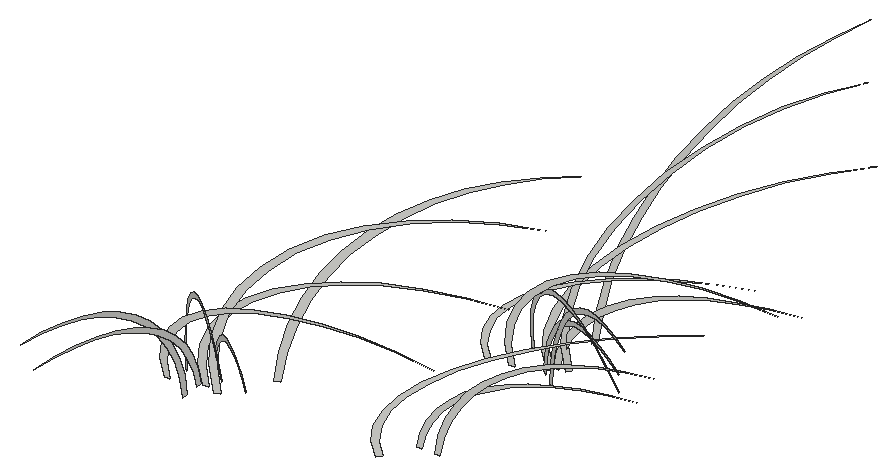
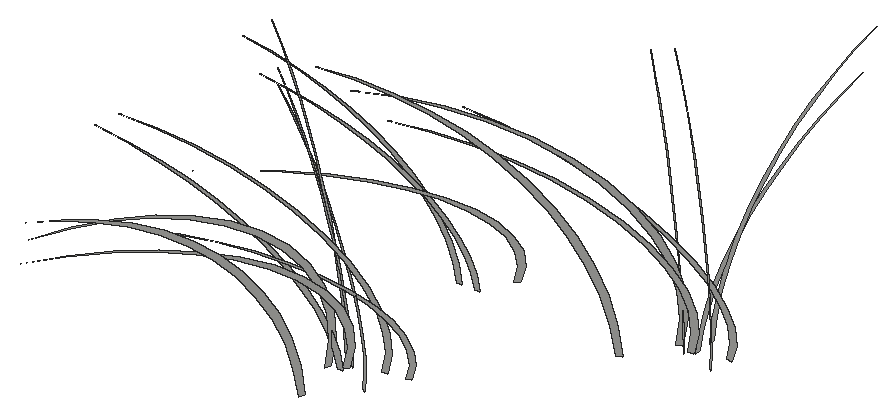
# SketchUp Ruby script. Lengths in inches.
U = 1.inch
M = Sketchup.active_model
def pt(a) = Geom::Point3d.new(a.map { |v| v * U })
def face(e, loops, mat)
  f = e.add_face(loops[0].map { |a| pt(a) })
  loops[1..].each { |l| e.add_face(l.map { |a| pt(a) }).erase! }
  f.material = f.back_material = mat if mat
  f
end
# faces: each face lists its corners as indices into pts; further lists are holes
def faces(e, pts, list, mat = nil) = list.each { |f| face(e, (f[0].is_a?(Array) ? f : [f]).map { |l| l.map { |i| pts[i] } }, mat) }
# xy, xz, yz: faces in a plane at the given z, y or x. An outline is a flat list of corners, or four numbers for a rectangle; further outlines are holes
def ring(l) = l.size == 4 ? [[l[0], l[1]], [l[2], l[1]], [l[2], l[3]], [l[0], l[3]]] : l.each_slice(2).to_a
def flat(e, list, mat, &to3) = list.each { |f| face(e, (f[0].is_a?(Array) ? f : [f]).map { |l| ring(l).map { |u, v| to3.(u, v) } }, mat) }
def xy(e, z, list, mat = nil) = flat(e, list, mat) { |x, y| [x, y, z] }
def xz(e, y, list, mat = nil) = flat(e, list, mat) { |x, z| [x, y, z] }
def yz(e, x, list, mat = nil) = flat(e, list, mat) { |y, z| [x, y, z] }
def lines(e, pts, list) = list.each { |a, b| e.add_line(pt(pts[a]), pt(pts[b])) }
# prism: a flat outline (further loops are holes) pulled along v
def prism(e, loops, v, mat = nil)
  f = face(e, loops, mat); d = Geom::Vector3d.new(v.map { |x| x * U })
  f.pushpull(f.normal.samedirection?(d) ? d.length : -d.length)
end
def box(e, o, s, mat = nil) = prism(e, [[o, [o[0] + s[0], o[1], o[2]], [o[0] + s[0], o[1] + s[1], o[2]], [o[0], o[1] + s[1], o[2]]]], [0, 0, s[2]], mat)
def at(x, y, z, deg = 0) = Geom::Transformation.translation(pt([x, y, z])) * Geom::Transformation.rotation(ORIGIN, Z_AXIS, deg.degrees)
def axes(o, x, y, z) = Geom::Transformation.new([*x, 0, *y, 0, *z, 0, *pt(o).to_a, 1])
def part(name) = M.definitions.add(name)
# library, detail: a bought-in or finely detailed component or shape, given as its bounding box
def library(name, o, s) = part(name).tap { |d| box(d.entities, o, s) }
def detail(e, o, s) = box(e.add_group.entities, o, s)
def put(e, d, t, mat = nil) = e.add_instance(d, t).tap { |i| i.material = mat if mat }
def group(e, t, mat = nil) = e.add_group.tap { |g| g.transformation = t; g.material = mat if mat }.entities
root = M.entities
g1 = group(root,at(14.6,754.69,-58.625))
p = [[0.6,-0.05,0],[0.27,-0.02,0],[0,0,0.91],[0.11,-0.01,1.82],[0.59,-0.05,2.72],[1.4375,-0.12,3.57],
  [2.62,-0.21,4.37],[4.12,-0.33,5.08],[5.89,-0.48,5.69],[7.89,-0.64,6.19],[10.08,-0.81,6.57],[12.39,-1,6.81],
  [14.77,-1.19,6.91],[17.16,-1.39,6.86],[14.8125,-1.2,6.87],[12.49,-1.01,6.74],[10.25,-0.83,6.48],[8.13,-0.66,6.09],
  [6.19,-0.5,5.59],[4.48,-0.36,4.98],[3.02,-0.24,4.28],[1.86,-0.15,3.5],[1.03,-0.08,2.66],[0.53,-0.04,1.79],
  [0.39,-0.03,0.89]]
faces(g1,p,[[0,1,2,3,4,5,6,7,8,9,10,11,12,13,14,15,16,17,18,19,20,21,22,23,24]])
g2 = group(root,at(28.83,766.22,-58.625))
p = [[0.22,0.52,0],[0.1,0.23,0],[0,0,1.44],[0.04,0.09,2.9],[0.21,0.51,4.32],[0.51,1.24,5.68],
  [0.93,2.26,6.95],[1.47,3.56,8.08],[2.1,5.09,9.06],[2.8125,6.82,9.85],[3.59,8.71,10.45],[4.41,10.7,10.83],
  [5.26,12.76,10.99],[6.11,14.82,10.91],[5.28,12.8,10.93],[4.45,10.79,10.72],[3.65,8.85,10.3125],[2.9,7.02,9.7],
  [2.2,5.35,8.89],[1.59,3.87,7.92],[1.08,2.61,6.8],[0.66,1.61,5.57],[0.37,0.89,4.23],[0.1875,0.46,2.84],
  [0.14,0.34,1.42]]
faces(g2,p,[[0,1,2,3,4,5,6,7,8,9,10,11,12,13,14,15,16,17,18,19,20,21,22,23,24]])
g3 = group(root,at(28.03,765.8125,-58.625))
p = [[0.32,0.47,0],[0.14,0.21,0],[0,0,1.07],[0.06,0.08,2.14],[0.31,0.46,3.2],[0.75,1.11,4.2],
  [1.37,2.03,5.14],[2.15,3.19,5.98],[3.08,4.5625,6.7],[4.13,6.11,7.29],[5.27,7.81,7.73],[6.48,9.59,8.01],
  [7.72,11.4375,8.125],[8.97,13.29,8.07],[7.75,11.47,8.08],[6.53,9.67,7.93],[5.36,7.9375,7.625],[4.25,6.3,7.17],
  [3.24,4.8,6.58],[2.34,3.47,5.86],[1.58,2.34,5.03],[0.97,1.44,4.12],[0.54,0.8,3.13],[0.28,0.41,2.1],
  [0.2,0.3,1.05]]
faces(g3,p,[[0,1,2,3,4,5,6,7,8,9,10,11,12,13,14,15,16,17,18,19,20,21,22,23,24]])
g4 = group(root,at(26.21,765.41,-58.625))
p = [[0.5625,0,0],[0.25,0,0],[0,0,1.07],[0.1,0,2.14],[0.55,0,3.2],[1.34,-0.01,4.2],
  [2.45,-0.01,5.14],[3.85,-0.02,5.98],[5.5,-0.03,6.7],[7.375,-0.04,7.29],[9.42,-0.05,7.73],[11.58,-0.06,8.01],
  [13.8,-0.08,8.125],[16.03,-0.09,8.07],[13.84,-0.08,8.08],[11.67,-0.07,7.93],[9.57,-0.05,7.625],[7.6,-0.04,7.17],
  [5.79,-0.03,6.58],[4.18,-0.02,5.86],[2.82,-0.02,5.03],[1.74,-0.01,4.12],[0.96,-0.01,3.13],[0.5,0,2.1],
  [0.36,0,1.05]]
faces(g4,p,[[0,1,2,3,4,5,6,7,8,9,10,11,12,13,14,15,16,17,18,19,20,21,22,23,24]])
g5 = group(root,at(28.22,766.44,-58.625))
p = [[12.67,-0.07,7.55],[14.59,-0.08,7.75],[12.73,-0.07,7.51],[10.95,-0.0625,7.17],[9.24,-0.05,6.75],[7.64,-0.04,6.24],
  [6.15,-0.03,5.66],[4.81,-0.03,5],[3.62,-0.02,4.28],[2.59,-0.01,3.5],[1.74,-0.01,2.67],[1.07,-0.01,1.81],
  [0.6,0,0.91],[0.33,0,0],[0,0,0],[0.22,0,0.93],[0.66,0,1.85],[1.32,-0.01,2.74],
  [2.17,-0.01,3.58],[3.22,-0.02,4.38],[4.45,-0.02,5.11],[5.85,-0.03,5.77],[7.38,-0.04,6.35],[9.05,-0.05,6.85],
  [10.82,-0.0625,7.25]]
faces(g5,p,[[0,1,2,3,4,5,6,7,8,9,10,11,12,13,14,15,16,17,18,19,20,21,22,23,24]])
g6 = group(root,at(26.89,754.75,-58.625))
p = [[0.41,0.35,0],[0.18,0.15,0],[0,0,0.8],[0.07,0.0625,1.61],[0.4,0.34,2.4],[0.97,0.83,3.16],
  [1.77,1.51,3.86],[2.79,2.37,4.49],[3.98,3.39,5.04],[5.34,4.54,5.48],[6.82,5.8,5.8125],[8.38,7.125,6.02],
  [9.99,8.49,6.11],[11.6,9.87,6.07],[10.02,8.52,6.08],[8.45,7.18,5.97],[6.93,5.89,5.74],[5.5,4.68,5.39],
  [4.1875,3.5625,4.95],[3.03,2.57,4.41],[2.04,1.74,3.78],[1.26,1.07,3.1],[0.69,0.59,2.36],[0.36,0.31,1.58],
  [0.26,0.22,0.79]]
faces(g6,p,[[0,1,2,3,4,5,6,7,8,9,10,11,12,13,14,15,16,17,18,19,20,21,22,23,24]])
g7 = group(root,at(17.33,754.84,-58.625))
p = [[0.52,0.22,0],[0.23,0.1,0],[0,0,1.44],[0.09,0.04,2.9],[0.51,0.21,4.32],[1.24,0.52,5.68],
  [2.26,0.94,6.95],[3.55,1.48,8.08],[5.08,2.12,9.06],[6.81,2.83,9.85],[8.69,3.62,10.45],[10.6875,4.45,10.83],
  [12.74,5.3,10.99],[14.8,6.16,10.91],[12.78,5.32,10.93],[10.78,4.49,10.72],[8.84,3.68,10.3125],[7.01,2.92,9.7],
  [5.34,2.22,8.89],[3.86,1.61,7.92],[2.61,1.09,6.8],[1.61,0.67,5.57],[0.89,0.37,4.23],[0.46,0.19,2.84],
  [0.34,0.14,1.42]]
faces(g7,p,[[0,1,2,3,4,5,6,7,8,9,10,11,12,13,14,15,16,17,18,19,20,21,22,23,24]])
g8 = group(root,at(16.48,755.12,-58.625))
p = [[0.55,0.11,0],[0.25,0.05,0],[0,0,1.07],[0.1,0.02,2.14],[0.54,0.11,3.2],[1.32,0.26,4.2],
  [2.4,0.47,5.14],[3.78,0.73,5.98],[5.4,1.05,6.7],[7.24,1.4,7.29],[9.24,1.79,7.73],[11.36,2.2,8.01],
  [13.55,2.63,8.125],[15.74,3.05,8.07],[13.59,2.64,8.08],[11.46,2.22,7.93],[9.4,1.82,7.625],[7.46,1.45,7.17],
  [5.68,1.1,6.58],[4.11,0.8,5.86],[2.77,0.54,5.03],[1.71,0.33,4.12],[0.94,0.18,3.13],[0.49,0.09,2.1],
  [0.36,0.07,1.05]]
faces(g8,p,[[0,1,2,3,4,5,6,7,8,9,10,11,12,13,14,15,16,17,18,19,20,21,22,23,24]])
g9 = group(root,at(14.91,756.12,-58.625))
p = [[0.4,-0.4,0],[0.18,-0.18,0],[0,0,1.07],[0.07,-0.07,2.14],[0.39,-0.39,3.2],[0.94,-0.95,4.2],
  [1.72,-1.74,5.14],[2.71,-2.74,5.98],[3.87,-3.91,6.7],[5.1875,-5.25,7.29],[6.62,-6.7,7.73],[8.14,-8.23,8.01],
  [9.7,-9.8125,8.125],[11.27,-11.4,8.07],[9.73,-9.84,8.08],[8.21,-8.3,7.93],[6.73,-6.81,7.625],[5.34,-5.4,7.17],
  [4.07,-4.11,6.58],[2.94,-2.97,5.86],[1.99,-2.01,5.03],[1.22,-1.24,4.12],[0.67,-0.68,3.13],[0.35,-0.35,2.1],
  [0.26,-0.26,1.05]]
faces(g9,p,[[0,1,2,3,4,5,6,7,8,9,10,11,12,13,14,15,16,17,18,19,20,21,22,23,24]])
g10 = group(root,at(17.06,755.43,-58.625))
p = [[8.91,-9.01,7.55],[10.26,-10.37,7.75],[8.95,-9.05,7.51],[7.7,-7.78,7.17],[6.5,-6.57,6.75],[5.37,-5.43,6.24],
  [4.33,-4.375,5.66],[3.38,-3.42,5],[2.54,-2.57,4.28],[1.82,-1.84,3.5],[1.22,-1.24,2.67],[0.75,-0.76,1.81],
  [0.42,-0.43,0.91],[0.23,-0.23,0],[0,0,0],[0.16,-0.16,0.93],[0.47,-0.47,1.85],[0.93,-0.9375,2.74],
  [1.53,-1.55,3.58],[2.27,-2.29,4.38],[3.13,-3.17,5.11],[4.11,-4.16,5.77],[5.19,-5.25,6.35],[6.36,-6.44,6.85],
  [7.61,-7.69,7.25]]
faces(g10,p,[[0,1,2,3,4,5,6,7,8,9,10,11,12,13,14,15,16,17,18,19,20,21,22,23,24]])
g11 = group(root,at(28.1875,769.29,-58.625))
p = [[4.83,11.72,12.66],[5.56,13.49,12.99],[4.85,11.77,12.59],[4.17,10.12,12.03],[3.52,8.54,11.32],[2.91,7.0625,10.47],
  [2.35,5.69,9.49],[1.83,4.45,8.38],[1.38,3.34,7.17],[0.99,2.39,5.87],[0.66,1.61,4.48],[0.41,0.99,3.03],
  [0.23,0.56,1.53],[0.125,0.31,0],[0,0,0],[0.09,0.21,1.57],[0.25,0.61,3.1],[0.5,1.22,4.59],
  [0.83,2.01,6.01],[1.23,2.98,7.34],[1.7,4.12,8.57],[2.23,5.4,9.68],[2.8125,6.83,10.65],[3.45,8.37,11.48],
  [4.125,10,12.15]]
faces(g11,p,[[0,1,2,3,4,5,6,7,8,9,10,11,12,13,14,15,16,17,18,19,20,21,22,23,24]])
g12 = group(root,at(29.01,765.1875,-58.625))
p = [[10.01,-7.77,9.36],[11.52,-8.94,9.61],[10.06,-7.81,9.31],[8.65,-6.71,8.89],[7.3,-5.67,8.37],[6.03,-4.68,7.74],
  [4.86,-3.77,7.02],[3.8,-2.95,6.2],[2.86,-2.22,5.3],[2.04,-1.59,4.34],[1.37,-1.07,3.3125],[0.85,-0.66,2.24],
  [0.48,-0.37,1.13],[0.26,-0.2,0],[0,0,0],[0.18,-0.14,1.16],[0.52,-0.41,2.3],[1.04,-0.81,3.39],
  [1.72,-1.33,4.44],[2.55,-1.98,5.43],[3.52,-2.73,6.34],[4.62,-3.58,7.15],[5.83,-4.53,7.875],[7.15,-5.55,8.49],
  [8.55,-6.64,8.98]]
faces(g12,p,[[0,1,2,3,4,5,6,7,8,9,10,11,12,13,14,15,16,17,18,19,20,21,22,23,24]])
g13 = group(root,at(28.08,765.91,-58.625))
p = [[10.01,-7.77,7.55],[11.52,-8.94,7.75],[10.06,-7.81,7.51],[8.65,-6.71,7.17],[7.3,-5.67,6.75],[6.03,-4.68,6.24],
  [4.86,-3.77,5.66],[3.8,-2.95,5],[2.86,-2.22,4.28],[2.04,-1.59,3.5],[1.37,-1.07,2.67],[0.85,-0.66,1.81],
  [0.48,-0.37,0.91],[0.26,-0.2,0],[0,0,0],[0.18,-0.14,0.93],[0.52,-0.41,1.85],[1.04,-0.81,2.74],
  [1.72,-1.33,3.58],[2.55,-1.98,4.38],[3.52,-2.73,5.11],[4.62,-3.58,5.77],[5.83,-4.53,6.35],[7.15,-5.55,6.85],
  [8.55,-6.64,7.25]]
faces(g13,p,[[0,1,2,3,4,5,6,7,8,9,10,11,12,13,14,15,16,17,18,19,20,21,22,23,24]])
g14 = group(root,at(25.06,765.09,-58.625))
p = [[0.43,0.17,0],[0.19,0.07,0],[0,0,0.76],[0.08,0.03,1.52],[0.42,0.16,2.27],[1.03,0.39,2.98],
  [1.875,0.72,3.65],[2.95,1.13,4.24],[4.21,1.62,4.76],[5.65,2.17,5.17],[7.21,2.76,5.49],[8.86,3.4,5.6875],
  [10.57,4.05,5.77],[12.28,4.71,5.73],[10.6,4.0625,5.74],[8.9375,3.43,5.63],[7.33,2.8125,5.41],[5.82,2.23,5.09],
  [4.43,1.7,4.67],[3.2,1.23,4.16],[2.16,0.83,3.57],[1.33,0.51,2.92],[0.73,0.28,2.22],[0.38,0.15,1.49],
  [0.28,0.11,0.74]]
faces(g14,p,[[0,1,2,3,4,5,6,7,8,9,10,11,12,13,14,15,16,17,18,19,20,21,22,23,24]])
g15 = group(root,at(26.01,767.52,-58.625))
p = [[0.48,-0.37,0],[0.21,-0.16,0],[0,0,0.91],[0.09,-0.07,1.82],[0.47,-0.36,2.72],[1.14,-0.88,3.57],
  [2.08,-1.61,4.37],[3.26,-2.53,5.08],[4.67,-3.625,5.69],[6.26,-4.86,6.19],[7.99,-6.2,6.57],[9.82,-7.62,6.81],
  [11.7,-9.08,6.91],[13.6,-10.56,6.86],[11.74,-9.11,6.87],[9.9,-7.68,6.74],[8.12,-6.3,6.48],[6.44,-5,6.09],
  [4.91,-3.81,5.59],[3.55,-2.75,4.98],[2.39,-1.86,4.28],[1.48,-1.15,3.5],[0.8125,-0.63,2.66],[0.42,-0.33,1.79],
  [0.31,-0.24,0.89]]
faces(g15,p,[[0,1,2,3,4,5,6,7,8,9,10,11,12,13,14,15,16,17,18,19,20,21,22,23,24]])
g16 = group(root,at(29.01,756.75,-58.625))
p = [[11.22,-0.0625,8.28],[12.91,-0.07,8.5],[11.27,-0.0625,8.24],[9.6875,-0.05,7.87],[8.18,-0.05,7.41],[6.76,-0.04,6.85],
  [5.45,-0.03,6.21],[4.26,-0.02,5.49],[3.2,-0.02,4.69],[2.29,-0.01,3.84],[1.54,-0.01,2.93],[0.95,-0.01,1.98],
  [0.53,0,1],[0.29,0,0],[0,0,0],[0.2,0,1.03],[0.59,0,2.03],[1.17,-0.01,3],
  [1.92,-0.01,3.93],[2.85,-0.02,4.8],[3.94,-0.02,5.61],[5.17,-0.03,6.33],[6.54,-0.04,6.97],[8.01,-0.04,7.51],
  [9.58,-0.05,7.95]]
faces(g16,p,[[0,1,2,3,4,5,6,7,8,9,10,11,12,13,14,15,16,17,18,19,20,21,22,23,24]])
g17 = group(root,at(27.97,756.76,-58.625))
p = [[11.22,-0.0625,6.68],[12.91,-0.07,6.86],[11.27,-0.0625,6.64],[9.6875,-0.05,6.35],[8.18,-0.05,5.97],[6.76,-0.04,5.52],
  [5.45,-0.03,5.01],[4.26,-0.02,4.42],[3.2,-0.02,3.79],[2.29,-0.01,3.1],[1.54,-0.01,2.36],[0.95,-0.01,1.6],
  [0.53,0,0.81],[0.29,0,0],[0,0,0],[0.2,0,0.83],[0.59,0,1.64],[1.17,-0.01,2.42],
  [1.92,-0.01,3.17],[2.85,-0.02,3.875],[3.94,-0.02,4.52],[5.17,-0.03,5.11],[6.54,-0.04,5.62],[8.01,-0.04,6.06],
  [9.58,-0.05,6.41]]
faces(g17,p,[[0,1,2,3,4,5,6,7,8,9,10,11,12,13,14,15,16,17,18,19,20,21,22,23,24]])
g18 = group(root,at(19.05,757.47,-58.625))
p = [[11.7,4.87,12.66],[13.47,5.61,12.99],[11.76,4.89,12.59],[10.11,4.21,12.03],[8.53,3.55,11.32],[7.05,2.94,10.47],
  [5.68,2.37,9.49],[4.44,1.85,8.38],[3.34,1.39,7.17],[2.39,0.99,5.87],[1.6,0.67,4.48],[0.99,0.41,3.03],
  [0.56,0.23,1.53],[0.3,0.125,0],[0,0,0],[0.21,0.09,1.57],[0.61,0.26,3.1],[1.22,0.51,4.59],
  [2.01,0.84,6.01],[2.98,1.24,7.34],[4.11,1.71,8.57],[5.4,2.25,9.68],[6.82,2.84,10.65],[8.36,3.48,11.48],
  [9.99,4.16,12.15]]
faces(g18,p,[[0,1,2,3,4,5,6,7,8,9,10,11,12,13,14,15,16,17,18,19,20,21,22,23,24]])
g19 = group(root,at(16.73,753.98,-58.625))
p = [[1.58,-12.57,9.36],[1.82,-14.47,9.61],[1.59,-12.63,9.31],[1.37,-10.86,8.89],[1.15,-9.17,8.37],[0.95,-7.58,7.74],
  [0.77,-6.11,7.02],[0.6,-4.77,6.2],[0.45,-3.59,5.3],[0.32,-2.57,4.34],[0.22,-1.72,3.3125],[0.13,-1.0625,2.24],
  [0.08,-0.6,1.13],[0.04,-0.33,0],[0,0,0],[0.03,-0.22,1.16],[0.08,-0.66,2.3],[0.16,-1.31,3.39],
  [0.27,-2.16,4.44],[0.4,-3.2,5.43],[0.56,-4.42,6.34],[0.73,-5.8,7.15],[0.92,-7.33,7.875],[1.13,-8.98,8.49],
  [1.35,-10.74,8.98]]
faces(g19,p,[[0,1,2,3,4,5,6,7,8,9,10,11,12,13,14,15,16,17,18,19,20,21,22,23,24]])
g20 = group(root,at(16.59,755.15,-58.625))
p = [[1.58,-12.57,7.55],[1.82,-14.47,7.75],[1.59,-12.63,7.51],[1.37,-10.86,7.17],[1.15,-9.17,6.75],[0.95,-7.58,6.24],
  [0.77,-6.11,5.66],[0.6,-4.77,5],[0.45,-3.59,4.28],[0.32,-2.57,3.5],[0.22,-1.72,2.67],[0.13,-1.0625,1.81],
  [0.08,-0.6,0.91],[0.04,-0.33,0],[0,0,0],[0.03,-0.22,0.93],[0.08,-0.66,1.85],[0.16,-1.31,2.74],
  [0.27,-2.16,3.58],[0.4,-3.2,4.38],[0.56,-4.42,5.11],[0.73,-5.8,5.77],[0.92,-7.33,6.35],[1.13,-8.98,6.85],
  [1.35,-10.74,7.25]]
faces(g20,p,[[0,1,2,3,4,5,6,7,8,9,10,11,12,13,14,15,16,17,18,19,20,21,22,23,24]])
